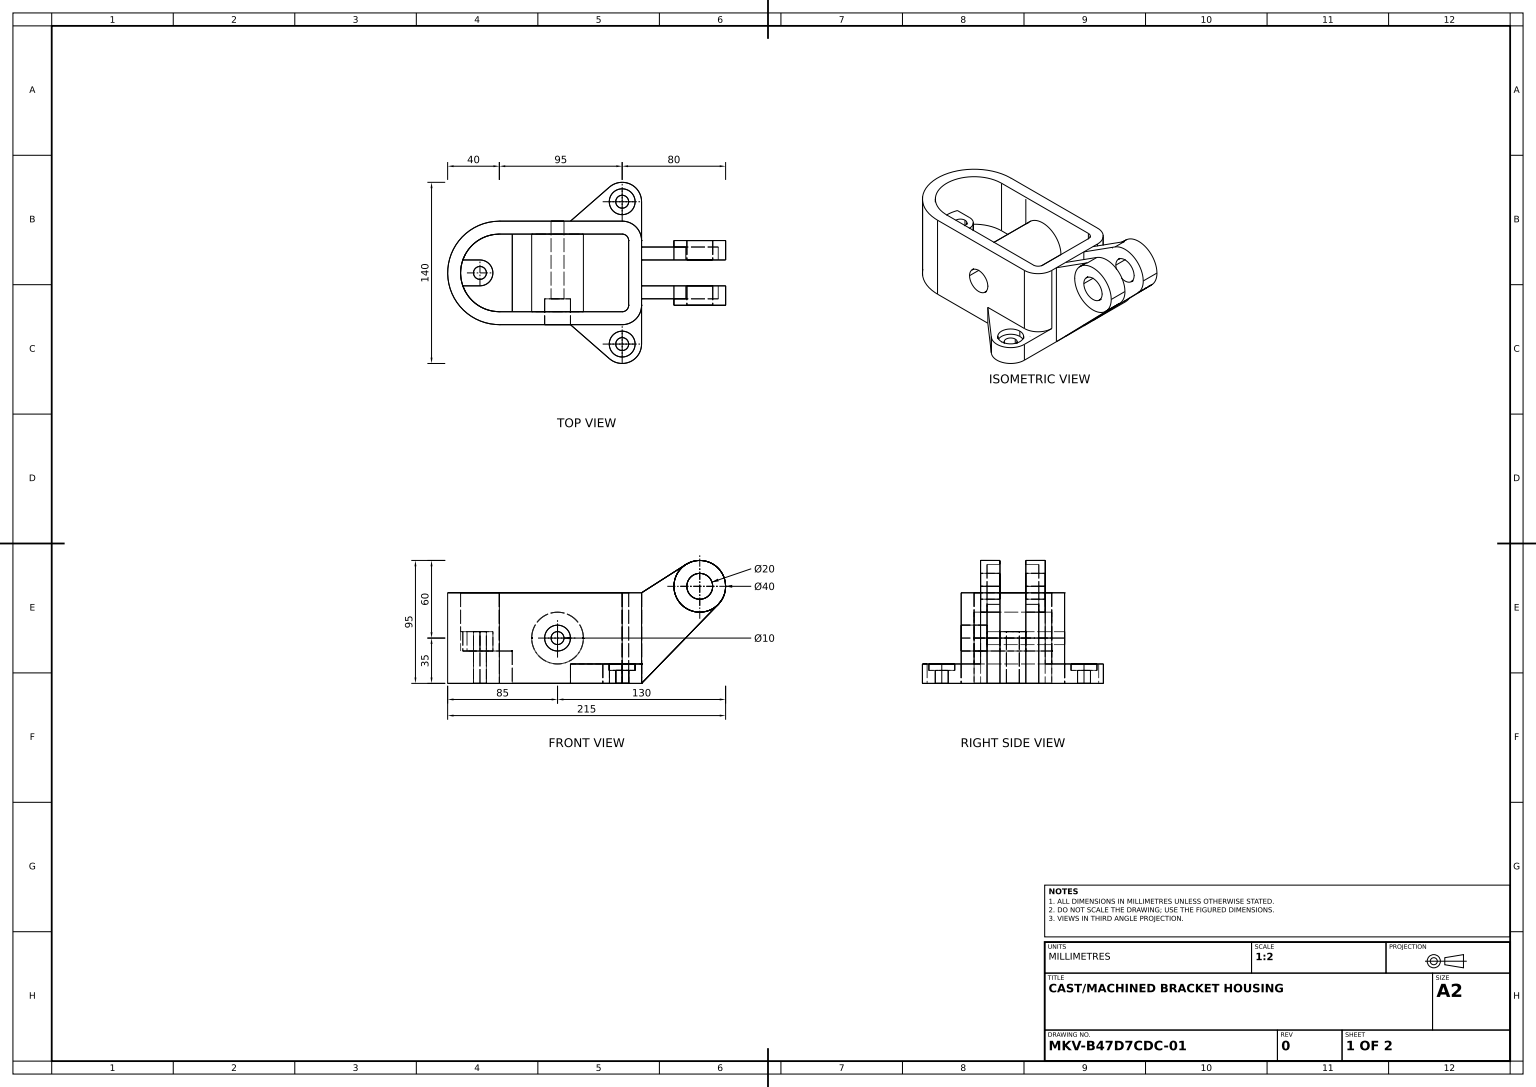
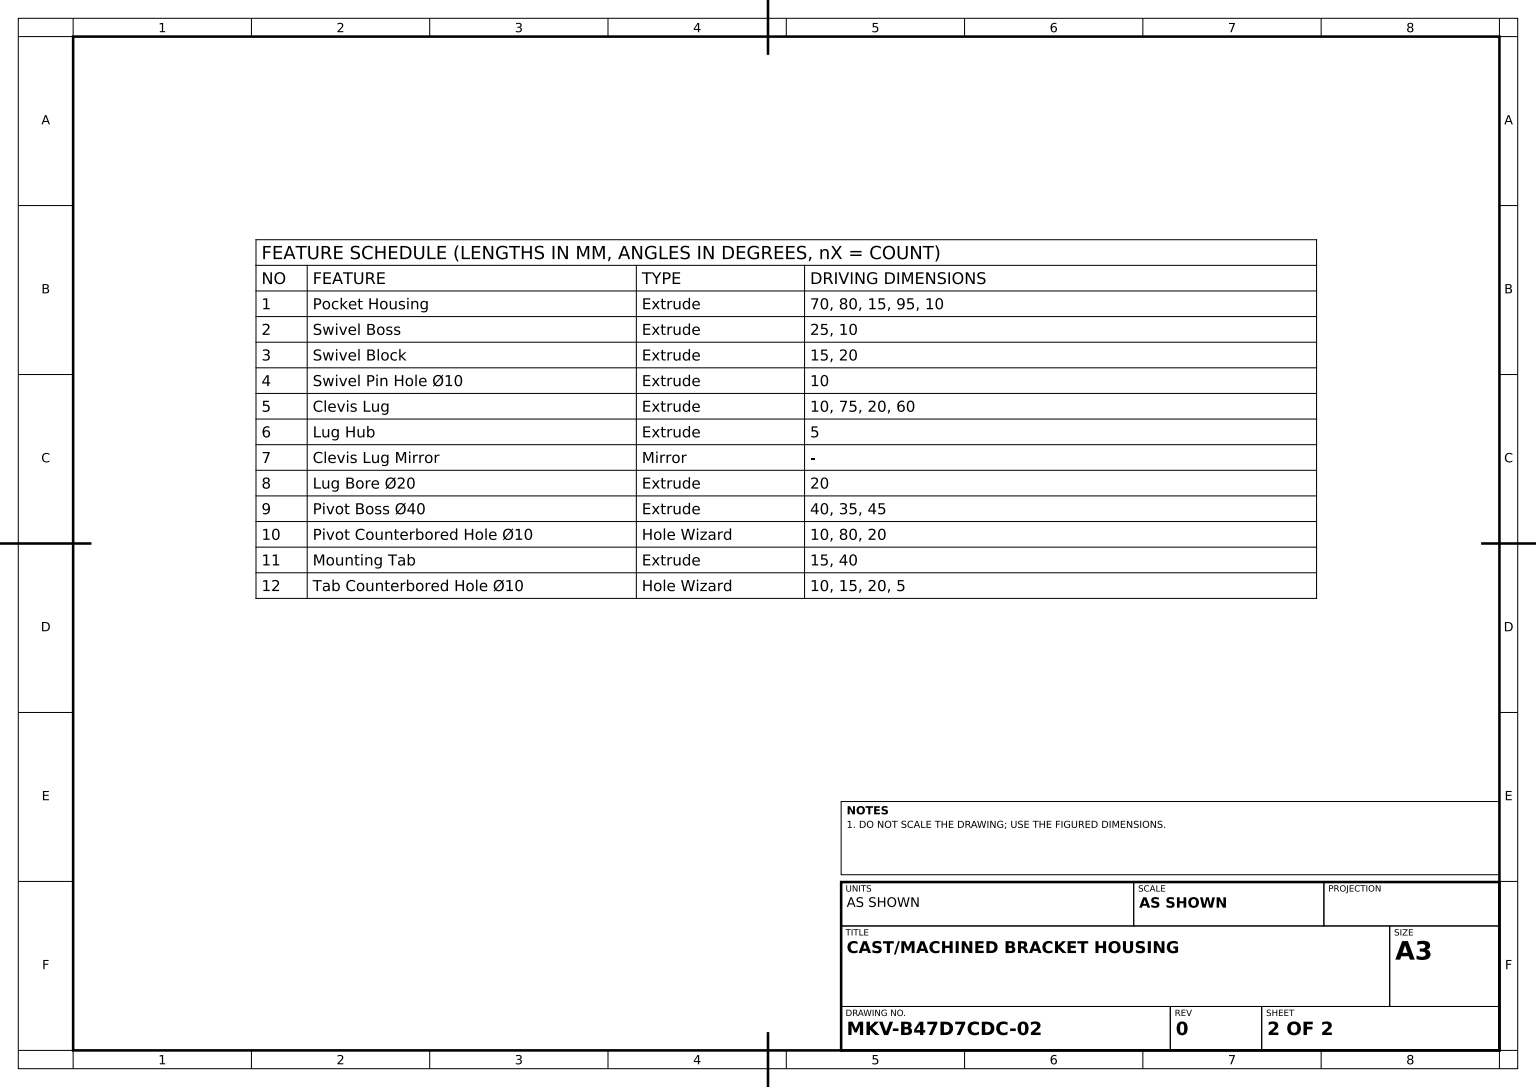
solid
v1 (25,75,-25)
v2 (25,75,-20)
e1 v1 v2 LINE
v3 (65,75,-25)
e2 v1 v3 CIRCLE(AX(P(45,75,-25),D(0,0,1),D(1,0,0)),20)
v4 (65,75,-10)
e3 v3 v4 LINE
v5 (59.342536,61.061145,-10)
e4 v5 v4 CIRCLE(AX(P(45,75,-10),D(0,0,1),D(1,0,0)),20)
v6 (59.342536,61.061145,-20)
e5 v6 v5 LINE
e6 v2 v6 CIRCLE(AX(P(45,75,-20),D(0,0,1),D(1,0,0)),20)
face CYL(AX(P(45,75,-20),D(0,0,1),D(1,0,0)),20) [-e1 e2 e3 -e4 -e5 -e6]
v7 (-55,0,40)
v8 (-24.863014,0,66.30137)
e7 v7 v8 LINE
v9 (-24.863014,15,66.30137)
e8 v9 v8 LINE
v10 (-55,15,40)
e9 v10 v9 LINE
e10 v10 v7 LINE
face PLANE(AX(P(-24.863014,15,66.30137),D(0.657534247,0,-0.753424658),D(-0.753424658,0,-0.657534247))) rev [e7 -e8 -e9 e10]
v11 (-125,0,-5)
v12 (-125,40,-5)
e11 v11 v12 LINE
v13 (-125,40,5)
e12 v12 v13 CIRCLE(AX(P(-125,40,0),D(0,1,0),D(0,0,1)),5)
v14 (-125,0,5)
e13 v14 v13 LINE
e14 v11 v14 CIRCLE(AX(P(-125,0,0),D(0,1,0),D(0,0,1)),5)
face CYL(AX(P(-125,0,0),D(0,1,0),D(0,0,1)),5) rev [e11 e12 -e13 -e14]
v15 (34.238039,91.857645,20)
v16 (0,70,20)
e15 v15 v16 LINE
v17 (0,0,20)
e16 v16 v17 LINE
v18 (59.342536,61.061145,20)
e17 v17 v18 LINE
v19 (25,75,20)
e18 v19 v18 CIRCLE(AX(P(45,75,20),D(0,0,1),D(1,0,0)),20)
e19 v15 v19 CIRCLE(AX(P(45,75,20),D(0,0,1),D(1,0,0)),20)
face PLANE(AX(P(45,75,20),D(0,0,1),D(1,0,0))) [e15 e16 e17 -e18 -e19]
v20 (0,15,55)
v21 (0,15,25)
e20 v20 v21 LINE
v22 (0,0,55)
e21 v20 v22 LINE
e22 v22 v17 LINE
v23 (0,70,25)
e23 v23 v16 LINE
e24 v23 v21 LINE
face PLANE(AX(P(0,70,0),D(-1,0,0),D(0,0,1))) rev [-e20 e21 e22 -e16 -e23 e24]
v24 (-15,10,-45)
v25 (-15,10,-65)
e25 v24 v25 CIRCLE(AX(P(-15,10,-55),D(0,1,0),D(0,0,1)),10)
e26 v25 v24 CIRCLE(AX(P(-15,10,-55),D(0,1,0),D(0,0,1)),10)
v26 (-15,10,-50)
v27 (-15,10,-60)
e27 v26 v27 CIRCLE(AX(P(-15,10,-55),D(0,1,0),D(0,0,1)),5)
e28 v27 v26 CIRCLE(AX(P(-15,10,-55),D(0,1,0),D(0,0,1)),5)
face PLANE(AX(P(-10,10,-55),D(0,-1,0),D(0,0,-1))) rev [e25 e26] [-e27 -e28]
v28 (-75,35,40)
v29 (-55,35,40)
e29 v28 v29 CIRCLE(AX(P(-65,35,40),D(0,0,1),D(1,0,0)),10)
e30 v29 v28 CIRCLE(AX(P(-65,35,40),D(0,0,1),D(1,0,0)),10)
v30 (-15,70,40)
v31 (-15,15,40)
e31 v30 v31 LINE
v32 (-110,70,40)
e32 v32 v30 LINE
v33 (-110,0,40)
e33 v32 v33 LINE
e34 v33 v7 LINE
e35 v31 v10 LINE
face PLANE(AX(P(-110,70,40),D(0,0,-1),D(-1,0,0))) rev [-e29 -e30] [-e31 -e32 e33 e34 -e10 -e35]
v34 (59.342536,61.061145,10)
e36 v18 v34 LINE
v35 (65,75,10)
e37 v34 v35 CIRCLE(AX(P(45,75,10),D(0,0,1),D(1,0,0)),20)
v36 (65,75,25)
e38 v36 v35 LINE
v37 (25,75,25)
e39 v37 v36 CIRCLE(AX(P(45,75,25),D(0,0,1),D(1,0,0)),20)
e40 v37 v19 LINE
face CYL(AX(P(45,75,20),D(0,0,-1),D(-1,0,0)),20) [e18 e36 e37 -e38 -e39 e40]
v38 (-10,70,-25)
v39 (-15,70,-30)
e41 v38 v39 CIRCLE(AX(P(-15,70,-25),D(0,1,0),D(0,0,1)),5)
v40 (-15,0,-30)
e42 v39 v40 LINE
v41 (-10,0,-25)
e43 v41 v40 CIRCLE(AX(P(-15,0,-25),D(0,1,0),D(0,0,1)),5)
e44 v38 v41 LINE
face CYL(AX(P(-15,70,-25),D(0,-1,0),D(0,0,-1)),5) rev [e41 e42 -e43 -e44]
v42 (0,70,-20)
v43 (0,70,-25)
e45 v42 v43 LINE
v44 (-15,70,-40)
e46 v43 v44 CIRCLE(AX(P(-15,70,-25),D(0,1,0),D(0,0,1)),15)
v45 (-110,70,-40)
e47 v44 v45 LINE
e48 v45 v32 CIRCLE(AX(P(-110,70,0),D(0,1,0),D(0,0,1)),40)
e49 v30 v23 CIRCLE(AX(P(-15,70,25),D(0,1,0),D(0,0,1)),15)
v46 (0,70,10)
e50 v16 v46 LINE
v47 (0,70,-10)
e51 v46 v47 LINE
e52 v42 v47 LINE
v48 (-15,70,30)
v49 (-10,70,25)
e53 v48 v49 CIRCLE(AX(P(-15,70,25),D(0,1,0),D(0,0,1)),5)
v50 (-110,70,30)
e54 v50 v48 LINE
v51 (-110,70,-30)
e55 v51 v50 CIRCLE(AX(P(-110,70,0),D(0,1,0),D(0,0,1)),30)
e56 v39 v51 LINE
e57 v49 v38 LINE
face PLANE(AX(P(-15,70,-25),D(0,1,0),D(0,0,1))) [e45 e46 e47 e48 e32 e49 e23 e50 e51 -e52] [-e53 -e54 -e55 -e56 -e41 -e57]
v52 (0,0,-20)
e58 v42 v52 LINE
v53 (34.238039,91.857645,-20)
e59 v53 v42 LINE
e60 v53 v2 CIRCLE(AX(P(45,75,-20),D(0,0,1),D(1,0,0)),20)
e61 v52 v6 LINE
face PLANE(AX(P(45,75,-20),D(0,0,-1),D(1,0,0))) [-e58 -e59 e60 e6 -e61]
v54 (34.238039,91.857645,-10)
e62 v53 v54 LINE
e63 v4 v54 CIRCLE(AX(P(45,75,-10),D(0,0,1),D(1,0,0)),20)
e64 v3 v1 CIRCLE(AX(P(45,75,-25),D(0,0,1),D(1,0,0)),20)
face CYL(AX(P(45,75,-20),D(0,0,1),D(1,0,0)),20) [e62 -e63 -e3 e64 e1 -e60]
v55 (-45,35,30)
v56 (-85,35,30)
e65 v55 v56 CIRCLE(AX(P(-65,35,30),D(0,0,-1),D(-1,0,0)),20)
v57 (-85,35,-30)
e66 v57 v56 LINE
v58 (-45,35,-30)
e67 v57 v58 CIRCLE(AX(P(-65,35,-30),D(0,0,1),D(1,0,0)),20)
e68 v58 v55 LINE
face CYL(AX(P(-65,35,-96.568542),D(0,0,1),D(1,0,0)),20) [e65 -e66 e67 e68]
v59 (-100,0,30)
v60 (-100,0,-30)
e69 v59 v60 LINE
v61 (-100,25,-30)
e70 v61 v60 LINE
v62 (-100,25,30)
e71 v62 v61 LINE
e72 v62 v59 LINE
face PLANE(AX(P(-100,25,-30),D(-1,0,0),D(0,0,1))) rev [e69 -e70 -e71 e72]
v63 (-15,15,-70)
v64 (-15,0,-70)
e73 v63 v64 LINE
v65 (0,15,-55)
e74 v65 v63 CIRCLE(AX(P(-15,15,-55),D(0,1,0),D(0,0,1)),15)
v66 (0,0,-55)
e75 v65 v66 LINE
e76 v66 v64 CIRCLE(AX(P(-15,0,-55),D(0,1,0),D(0,0,1)),15)
face CYL(AX(P(-15,15,-55),D(0,-1,0),D(0,0,-1)),15) [-e73 -e74 e75 e76]
v67 (-55,0,-40)
v68 (-110,0,-40)
e77 v67 v68 LINE
v69 (-24.863014,0,-66.30137)
e78 v69 v67 LINE
e79 v64 v69 CIRCLE(AX(P(-15,0,-55),D(0,1,0),D(0,0,1)),15)
e80 v52 v66 LINE
v70 (0,0,-10)
e81 v52 v70 LINE
v71 (0,0,10)
e82 v71 v70 LINE
e83 v17 v71 LINE
e84 v8 v22 CIRCLE(AX(P(-15,0,55),D(0,1,0),D(0,0,-1)),15)
e85 v68 v33 CIRCLE(AX(P(-110,0,0),D(0,1,0),D(0,0,1)),40)
e86 v14 v11 CIRCLE(AX(P(-125,0,0),D(0,1,0),D(0,0,1)),5)
v72 (-15,0,-60)
v73 (-15,0,-50)
e87 v72 v73 CIRCLE(AX(P(-15,0,-55),D(0,1,0),D(0,0,1)),5)
e88 v73 v72 CIRCLE(AX(P(-15,0,-55),D(0,1,0),D(0,0,1)),5)
v74 (-15,0,60)
v75 (-15,0,50)
e89 v74 v75 CIRCLE(AX(P(-15,0,55),D(0,1,0),D(0,0,1)),5)
e90 v75 v74 CIRCLE(AX(P(-15,0,55),D(0,1,0),D(0,0,1)),5)
v76 (-10,0,25)
e91 v76 v41 LINE
e92 v40 v60 LINE
v77 (-15,0,30)
e93 v59 v77 LINE
e94 v77 v76 CIRCLE(AX(P(-15,0,25),D(0,1,0),D(0,0,1)),5)
face PLANE(AX(P(-15,0,-25),D(0,1,0),D(0,0,1))) rev [-e77 -e78 -e79 -e76 -e80 e81 -e82 -e83 -e22 -e84 -e7 -e34 -e85] [e14 e86] [e87 e88] [e89 e90] [e91 e43 e92 -e69 e93 e94]
e95 v13 v12 CIRCLE(AX(P(-125,40,0),D(0,1,0),D(0,0,1)),5)
v78 (-138.284271,40,-10)
v79 (-138.284271,40,10)
e96 v78 v79 CIRCLE(AX(P(-110,40,0),D(0,1,0),D(0,0,1)),30)
v80 (-125,40,10)
e97 v79 v80 LINE
v81 (-125,40,-10)
e98 v80 v81 CIRCLE(AX(P(-125,40,0),D(0,1,0),D(0,0,1)),10)
e99 v81 v78 LINE
face PLANE(AX(P(-125,40,0),D(0,1,0),D(0,0,1))) [-e12 -e95] [e96 e97 e98 e99]
e100 v49 v76 LINE
e101 v48 v77 LINE
face CYL(AX(P(-15,70,25),D(0,-1,0),D(0,0,-1)),5) rev [e100 -e94 -e101 e53]
e102 v54 v47 LINE
face PLANE(AX(P(0,70,-20),D(-0.538098029,0.842882264,0),D(-0.842882264,-0.538098029,0))) [e59 e52 -e102 -e62]
v82 (-75,35,20)
v83 (-55,35,20)
e103 v82 v83 CIRCLE(AX(P(-65,35,20),D(0,0,1),D(1,0,0)),10)
e104 v82 v28 LINE
e105 v83 v29 LINE
face CYL(AX(P(-65,35,40),D(0,0,1),D(1,0,0)),10) rev [-e103 e104 e29 -e105]
v84 (-110,25,-30)
e106 v51 v84 LINE
e107 v61 v84 LINE
e108 v58 v57 CIRCLE(AX(P(-65,35,-30),D(0,0,1),D(1,0,0)),20)
face PLANE(AX(P(-15,70,-30),D(0,0,1),D(1,0,0))) [-e42 e56 e106 -e107 e70 -e92] [-e67 -e108]
v85 (-138.284271,25,-10)
e109 v84 v85 CIRCLE(AX(P(-110,25,0),D(0,1,0),D(0,0,1)),30)
v86 (-125,25,-10)
e110 v86 v85 LINE
v87 (-125,25,10)
e111 v87 v86 CIRCLE(AX(P(-125,25,0),D(0,1,0),D(0,0,1)),10)
v88 (-138.284271,25,10)
e112 v88 v87 LINE
v89 (-110,25,30)
e113 v88 v89 CIRCLE(AX(P(-110,25,0),D(0,1,0),D(0,0,1)),30)
e114 v89 v62 LINE
face PLANE(AX(P(-110,25,0),D(0,1,0),D(0,0,1))) [e71 e107 e109 -e110 -e111 -e112 e113 e114]
v90 (35,75,10)
v91 (35,75,25)
e115 v90 v91 LINE
v92 (55,75,25)
e116 v91 v92 CIRCLE(AX(P(45,75,25),D(0,0,1),D(1,0,0)),10)
v93 (55,75,10)
e117 v93 v92 LINE
e118 v90 v93 CIRCLE(AX(P(45,75,10),D(0,0,1),D(1,0,0)),10)
face CYL(AX(P(45,75,-40),D(0,0,1),D(1,0,0)),10) rev [e115 e116 -e117 -e118]
v94 (34.238039,91.857645,10)
e119 v35 v94 CIRCLE(AX(P(45,75,10),D(0,0,1),D(1,0,0)),20)
e120 v15 v94 LINE
e121 v36 v37 CIRCLE(AX(P(45,75,25),D(0,0,1),D(1,0,0)),20)
face CYL(AX(P(45,75,20),D(0,0,-1),D(-1,0,0)),20) [e38 e119 -e120 e19 -e40 -e121]
v95 (-60,35,20)
v96 (-70,35,20)
e122 v95 v96 CIRCLE(AX(P(-65,35,20),D(0,0,1),D(1,0,0)),5)
v97 (-70,35,-40)
e123 v97 v96 LINE
v98 (-60,35,-40)
e124 v98 v97 CIRCLE(AX(P(-65,35,-40),D(0,0,1),D(1,0,0)),5)
e125 v98 v95 LINE
face CYL(AX(P(-65,35,40),D(0,0,1),D(1,0,0)),5) rev [e122 -e123 -e124 e125]
face PLANE(AX(P(-10,70,0),D(-1,0,0),D(0,0,1))) [-e91 -e100 e57 e44]
v99 (55,75,-25)
v100 (35,75,-25)
e126 v99 v100 CIRCLE(AX(P(45,75,-25),D(0,0,-1),D(-1,0,0)),10)
v101 (35,75,-10)
e127 v100 v101 LINE
v102 (55,75,-10)
e128 v102 v101 CIRCLE(AX(P(45,75,-10),D(0,0,-1),D(-1,0,0)),10)
e129 v99 v102 LINE
face CYL(AX(P(45,75,-40),D(0,0,1),D(1,0,0)),10) rev [e126 e127 -e128 -e129]
e130 v71 v34 LINE
e131 v46 v71 LINE
e132 v94 v46 LINE
e133 v93 v90 CIRCLE(AX(P(45,75,10),D(0,0,1),D(1,0,0)),10)
face PLANE(AX(P(45,75,10),D(0,0,1),D(1,0,0))) rev [-e119 -e37 -e130 -e131 -e132] [e118 e133]
e134 v9 v20 CIRCLE(AX(P(-15,15,55),D(0,1,0),D(0,0,-1)),15)
face CYL(AX(P(-15,15,55),D(0,-1,0),D(0,0,-1)),15) [e84 -e21 -e134 e8]
v103 (0,15,-25)
e135 v43 v103 LINE
v104 (-15,15,-40)
e136 v104 v103 CIRCLE(AX(P(-15,15,-25),D(0,-1,0),D(0,0,1)),15)
e137 v44 v104 LINE
face CYL(AX(P(-15,70,-25),D(0,-1,0),D(0,0,-1)),15) [e135 -e136 -e137 -e46]
e138 v92 v91 CIRCLE(AX(P(45,75,25),D(0,0,1),D(1,0,0)),10)
face PLANE(AX(P(45,75,25),D(0,0,1),D(1,0,0))) [e121 e39] [-e138 -e116]
e139 v103 v65 LINE
v105 (-24.863014,15,-66.30137)
e140 v63 v105 CIRCLE(AX(P(-15,15,-55),D(0,1,0),D(0,0,1)),15)
v106 (-55,15,-40)
e141 v105 v106 LINE
e142 v106 v104 LINE
v107 (-15,15,-65)
v108 (-15,15,-45)
e143 v107 v108 CIRCLE(AX(P(-15,15,-55),D(0,1,0),D(0,0,1)),10)
e144 v108 v107 CIRCLE(AX(P(-15,15,-55),D(0,1,0),D(0,0,1)),10)
face PLANE(AX(P(-15,15,-55),D(0,1,0),D(0,0,1))) [e139 e74 e140 e141 e142 e136] [-e143 -e144]
e145 v50 v89 LINE
e146 v56 v55 CIRCLE(AX(P(-65,35,30),D(0,0,-1),D(-1,0,0)),20)
face PLANE(AX(P(-110,70,30),D(0,0,-1),D(-1,0,0))) [e54 e101 -e93 -e72 -e114 -e145] [-e146 -e65]
v109 (-15,10,50)
e147 v75 v109 LINE
v110 (-15,10,60)
e148 v109 v110 CIRCLE(AX(P(-15,10,55),D(0,1,0),D(0,0,1)),5)
e149 v74 v110 LINE
face CYL(AX(P(-15,15,55),D(0,1,0),D(0,0,1)),5) rev [-e90 e147 e148 -e149]
v111 (-15,10,65)
v112 (-15,15,65)
e150 v111 v112 LINE
v113 (-15,10,45)
e151 v113 v111 CIRCLE(AX(P(-15,10,55),D(0,1,0),D(0,0,1)),10)
v114 (-15,15,45)
e152 v113 v114 LINE
e153 v114 v112 CIRCLE(AX(P(-15,15,55),D(0,1,0),D(0,0,1)),10)
face CYL(AX(P(-15,15,55),D(0,1,0),D(0,0,1)),10) rev [-e150 -e151 e152 e153]
face PLANE(AX(P(0,0,20),D(-0.717126783,0.696942736,0),D(-0.696942736,-0.717126783,0))) rev [e83 e130 -e36 -e17]
face CYL(AX(P(45,75,-40),D(0,0,1),D(1,0,0)),10) rev [-e115 -e133 e117 e138]
face CYL(AX(P(-125,0,0),D(0,1,0),D(0,0,1)),5) rev [-e86 e13 e95 -e11]
e154 v106 v67 LINE
e155 v105 v69 LINE
face PLANE(AX(P(-24.863014,15,-66.30137),D(0.657534247,0,0.753424658),D(0.753424658,0,-0.657534247))) rev [e78 -e154 -e141 e155]
face CYL(AX(P(-65,35,-96.568542),D(0,0,1),D(1,0,0)),20) [e146 -e68 e108 e66]
e156 v100 v99 CIRCLE(AX(P(45,75,-25),D(0,0,-1),D(-1,0,0)),10)
face PLANE(AX(P(45,75,-25),D(0,0,-1),D(1,0,0))) [-e126 -e156] [-e64 -e2]
e157 v21 v31 CIRCLE(AX(P(-15,15,25),D(0,-1,0),D(0,0,-1)),15)
e158 v112 v114 CIRCLE(AX(P(-15,15,55),D(0,1,0),D(0,0,1)),10)
face PLANE(AX(P(-15,15,55),D(0,-1,0),D(0,0,-1))) rev [e35 e9 e134 e20 e157] [-e153 -e158]
e159 v96 v95 CIRCLE(AX(P(-65,35,20),D(0,0,1),D(1,0,0)),5)
e160 v83 v82 CIRCLE(AX(P(-65,35,20),D(0,0,1),D(1,0,0)),10)
face PLANE(AX(P(-60,35,20),D(0,0,-1),D(-1,0,0))) rev [-e122 -e159] [e103 e160]
e161 v101 v102 CIRCLE(AX(P(45,75,-10),D(0,0,-1),D(-1,0,0)),10)
e162 v47 v70 LINE
e163 v70 v5 LINE
face PLANE(AX(P(45,75,-10),D(0,0,-1),D(1,0,0))) rev [e161 e128] [e162 e163 e4 e63 e102]
face PLANE(AX(P(0,70,20),D(0.538098029,-0.842882264,0),D(0.842882264,0.538098029,0))) rev [-e15 e120 e132 -e50]
face PLANE(AX(P(0,70,0),D(-1,0,0),D(0,0,1))) rev [-e162 -e51 e131 e82]
e164 v25 v107 LINE
e165 v24 v108 LINE
face CYL(AX(P(-15,15,-55),D(0,1,0),D(0,0,1)),10) rev [-e164 -e25 e165 e144]
e166 v110 v109 CIRCLE(AX(P(-15,10,55),D(0,1,0),D(0,0,1)),5)
face CYL(AX(P(-15,15,55),D(0,1,0),D(0,0,1)),5) rev [-e147 -e89 e149 e166]
e167 v79 v88 LINE
e168 v80 v87 LINE
face PLANE(AX(P(-125,40,10),D(0,0,-1),D(-1,0,0))) rev [-e97 e167 e112 -e168]
e169 v73 v26 LINE
e170 v72 v27 LINE
face CYL(AX(P(-15,15,-55),D(0,1,0),D(0,0,1)),5) rev [-e169 -e87 e170 e28]
face PLANE(AX(P(0,70,0),D(-1,0,0),D(0,0,1))) rev [-e75 -e139 -e135 -e45 e58 e80]
face CYL(AX(P(45,75,-40),D(0,0,1),D(1,0,0)),10) rev [e156 e129 -e161 -e127]
face PLANE(AX(P(0,0,-20),D(0.717126783,-0.696942736,0),D(0.696942736,0.717126783,0))) [-e163 -e81 e61 e5]
face CYL(AX(P(-15,15,-55),D(0,-1,0),D(0,0,-1)),15) [-e140 e73 e79 -e155]
e171 v97 v98 CIRCLE(AX(P(-65,35,-40),D(0,0,1),D(1,0,0)),5)
face CYL(AX(P(-65,35,40),D(0,0,1),D(1,0,0)),5) rev [e159 -e125 -e171 e123]
face CYL(AX(P(-15,15,-55),D(0,1,0),D(0,0,1)),10) rev [e164 e143 -e165 -e26]
face CYL(AX(P(-15,15,-55),D(0,1,0),D(0,0,1)),5) rev [-e170 -e88 e169 e27]
face CYL(AX(P(-65,35,40),D(0,0,1),D(1,0,0)),10) rev [e105 e30 -e104 -e160]
face CYL(AX(P(-15,70,25),D(0,-1,0),D(0,0,-1)),15) [e31 -e157 -e24 -e49]
e172 v45 v68 LINE
face CYL(AX(P(-110,70,0),D(0,-1,0),D(0,0,-1)),40) [-e48 e172 e85 -e33]
e173 v111 v113 CIRCLE(AX(P(-15,10,55),D(0,1,0),D(0,0,1)),10)
face CYL(AX(P(-15,15,55),D(0,1,0),D(0,0,1)),10) rev [e158 -e152 -e173 e150]
e174 v81 v86 LINE
e175 v78 v85 LINE
face PLANE(AX(P(-125,40,-10),D(0,0,1),D(1,0,0))) rev [e174 e110 -e175 -e99]
face PLANE(AX(P(-10,10,55),D(0,-1,0),D(0,0,-1))) rev [-e148 -e166] [e151 e173]
face CYL(AX(P(-125,40,0),D(0,-1,0),D(0,0,-1)),10) [-e174 -e98 e168 e111]
face PLANE(AX(P(-15,70,-40),D(0,0,1),D(1,0,0))) rev [e154 e77 -e172 -e47 e137 -e142] [e171 e124]
face CYL(AX(P(-110,70,0),D(0,-1,0),D(0,0,-1)),30) rev [-e96 e175 -e109 -e106 e55 e145 -e113 -e167]
